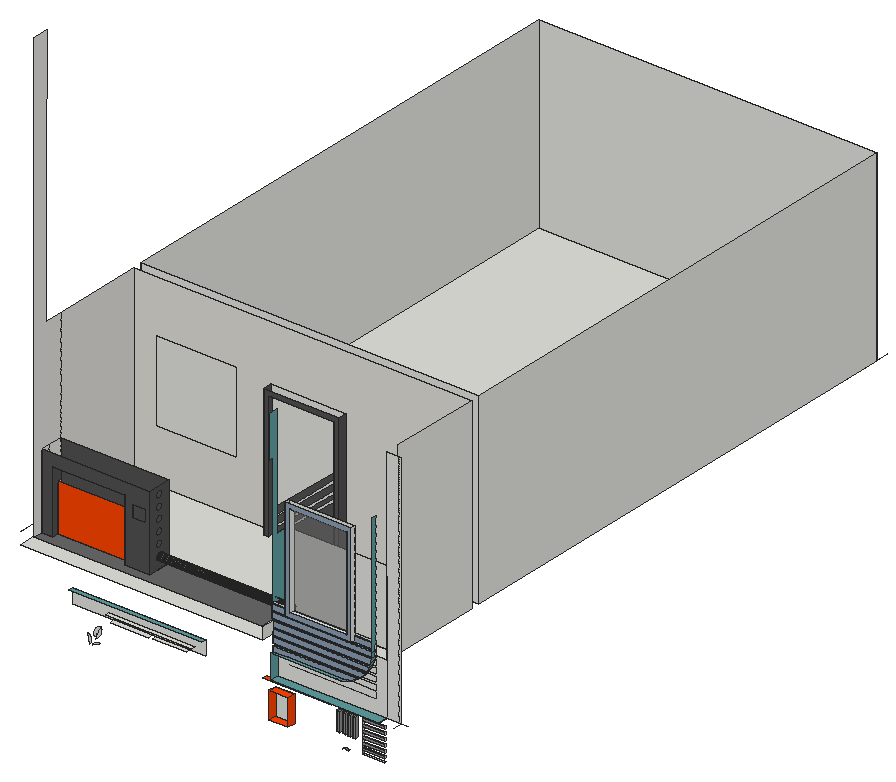
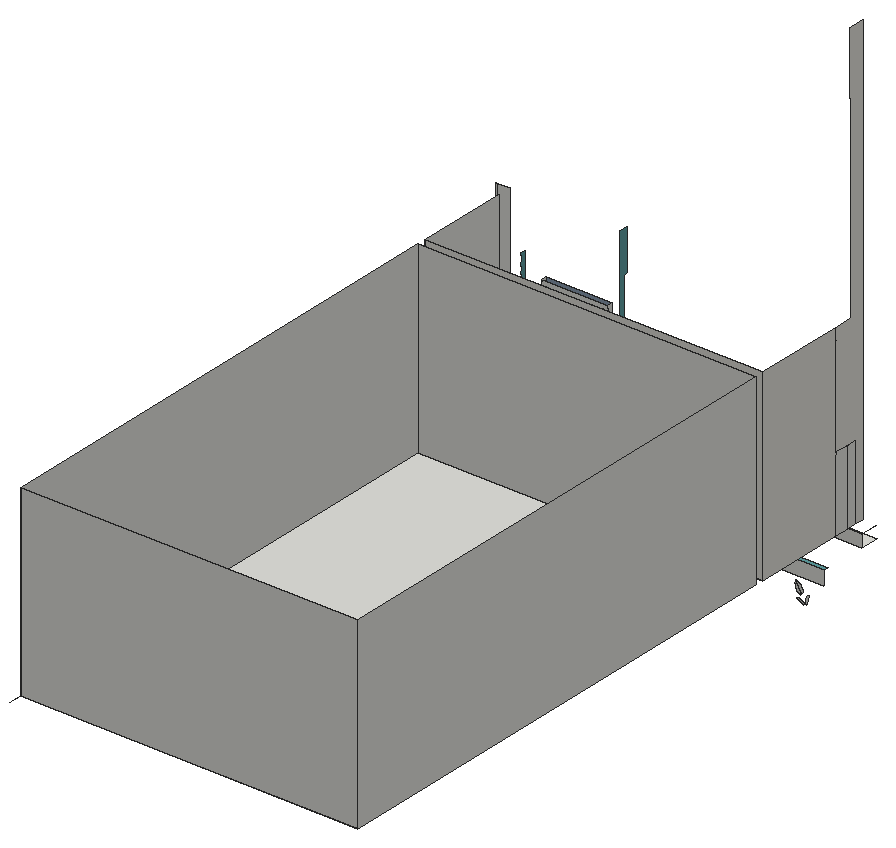
# SketchUp Ruby script. Lengths in inches.
U = 1.inch
M = Sketchup.active_model
def pt(a) = Geom::Point3d.new(a.map { |v| v * U })
def face(e, loops, mat)
  f = e.add_face(loops[0].map { |a| pt(a) })
  loops[1..].each { |l| e.add_face(l.map { |a| pt(a) }).erase! }
  f.material = f.back_material = mat if mat
  f
end
# faces: each face lists its corners as indices into pts; further lists are holes
def faces(e, pts, list, mat = nil) = list.each { |f| face(e, (f[0].is_a?(Array) ? f : [f]).map { |l| l.map { |i| pts[i] } }, mat) }
# xy, xz, yz: faces in a plane at the given z, y or x. An outline is a flat list of corners, or four numbers for a rectangle; further outlines are holes
def ring(l) = l.size == 4 ? [[l[0], l[1]], [l[2], l[1]], [l[2], l[3]], [l[0], l[3]]] : l.each_slice(2).to_a
def flat(e, list, mat, &to3) = list.each { |f| face(e, (f[0].is_a?(Array) ? f : [f]).map { |l| ring(l).map { |u, v| to3.(u, v) } }, mat) }
def xy(e, z, list, mat = nil) = flat(e, list, mat) { |x, y| [x, y, z] }
def xz(e, y, list, mat = nil) = flat(e, list, mat) { |x, z| [x, y, z] }
def yz(e, x, list, mat = nil) = flat(e, list, mat) { |y, z| [x, y, z] }
def lines(e, pts, list) = list.each { |a, b| e.add_line(pt(pts[a]), pt(pts[b])) }
# prism: a flat outline (further loops are holes) pulled along v
def prism(e, loops, v, mat = nil)
  f = face(e, loops, mat); d = Geom::Vector3d.new(v.map { |x| x * U })
  f.pushpull(f.normal.samedirection?(d) ? d.length : -d.length)
end
def box(e, o, s, mat = nil) = prism(e, [[o, [o[0] + s[0], o[1], o[2]], [o[0] + s[0], o[1] + s[1], o[2]], [o[0], o[1] + s[1], o[2]]]], [0, 0, s[2]], mat)
def at(x, y, z, deg = 0) = Geom::Transformation.translation(pt([x, y, z])) * Geom::Transformation.rotation(ORIGIN, Z_AXIS, deg.degrees)
def axes(o, x, y, z) = Geom::Transformation.new([*x, 0, *y, 0, *z, 0, *pt(o).to_a, 1])
def part(name) = M.definitions.add(name)
# library, detail: a bought-in or finely detailed component or shape, given as its bounding box
def library(name, o, s) = part(name).tap { |d| box(d.entities, o, s) }
def detail(e, o, s) = box(e.add_group.entities, o, s)
def put(e, d, t, mat = nil) = e.add_instance(d, t).tap { |i| i.material = mat if mat }
def group(e, t, mat = nil) = e.add_group.tap { |g| g.transformation = t; g.material = mat if mat }.entities
root = M.entities
M.materials.add("[0024_OrangeRed]").color = [255, 69, 0]
M.materials.add("[0081_CadetBlue]").color = [95, 158, 160]
M.materials.add("[0110_LightSlateGray]").color = [139, 158, 178]
M.materials.add("[0134_DimGray]").color = [105, 105, 105]
M.materials.add("[0135_DarkGray]").color = [81, 81, 81]
M.materials.add("[Color M04]").color = [142, 142, 142]
M.materials.add("[Marble Carrara Gold Floor Tile]").color = [225, 223, 217]
M.materials.add("[Translucent Glass Gray]").color = [128, 128, 128]
M.materials["[Translucent Glass Gray]"].alpha = 0.5
xy(root,61.1,[[216.37,11,230.7,12]])
xy(root,61.11,[[157.99,9,169.99,14.125]],"[0024_OrangeRed]")
xy(root,63.25,[[216.37,11,230.7,12]])
xy(root,64.54,[[216.37,11,230.7,12]])
xy(root,66.6875,[[216.37,11,230.7,12]])
xy(root,67.98,[[216.37,11,230.7,12]])
xy(root,69.76,[[211.55,9.125,213.55,11],[201.43,9.25,203.43,11],[204.8,9.25,206.8,11],[208.18,9.25,210.18,11]])
xy(root,70.125,[[216.37,11,230.7,12]])
xy(root,71.42,[[216.37,11,230.7,12]])
xy(root,73.5625,[[216.37,11,230.7,12]])
xy(root,74.85,[[216.37,11,230.7,12]])
xy(root,77,[[216.37,11,230.7,12]])
xy(root,78.23,[[157.99,9,169.99,14.125]],"[0024_OrangeRed]")
xy(root,78.29,[[216.37,11,230.7,12]])
xy(root,80.4375,[[216.37,11,230.7,12]])
xy(root,81.73,[[216.37,11,230.7,12]])
xy(root,81.89,[[211.55,9.125,213.55,11],[201.43,9.25,203.43,11],[204.8,9.25,206.8,11],[208.18,9.25,210.18,11]],"[Color M04]")
xy(root,83.5625,[[58.13,6,82.62,9],[85.26,6,107.11,9]])
xy(root,83.875,[[153.86,9,198.26,12]],"[0024_OrangeRed]")
xy(root,83.875,[[198.26,11,216.37,12]],"[Color M04]")
xy(root,86.5625,[[161.25,6,230.7,12]],"[0081_CadetBlue]")
xy(root,86.73,[[54.96,6,110.28,9]])
xy(root,90.99,[[29.19,9,114.82,12]],"[0081_CadetBlue]")
xy(root,102.07,[[161.25,6,203.39,9]],"[0081_CadetBlue]")
xy(root,102.24,[[161.25,8,170.69,9]])
xy(root,102.27,[[170.69,8,206.44,9]])
xy(root,105.62,[[161.25,8,215.65,9]],"[0110_LightSlateGray]")
xy(root,106.98,[[161.25,8,217.65,9]])
xy(root,110.36,[[161.25,8,221.11,9]],"[0110_LightSlateGray]")
xy(root,111.72,[[161.25,8,222.18,9]],"[0110_LightSlateGray]")
xy(root,112.3125,[[5,0,161.25,12]])
xy(root,115.1,[[161.25,8,224.19,9]],"[0110_LightSlateGray]")
xy(root,116.46,[[161.25,8,224.85,9]],"[0110_LightSlateGray]")
xy(root,116.6875,[[83.4375,12,160.53,21]])
xy(root,119.84,[[161.25,8,225.92,9]],"[0110_LightSlateGray]")
xy(root,120,[[160.53,0,161.25,9],[14,6,21.23,12],[67.5,6,83.4375,12],[160.53,9,161.25,12],[21.23,10.125,67.5,12],
  [14,12,83.4375,21],[160.53,12,231.375,21],[14,21,231.375,21,231.375,79.875,150.55,79.875,150.55,73.875,147.55,73.875,147.55,76.875,105.55,76.875,105.55,73.875,102.55,73.875,102.55,79.875,14,79.875],[102.55,73.875,105.55,73.875,105.55,76.875,147.55,76.875,147.55,73.875,150.55,73.875,150.55,79.875,102.55,79.875],[14,85.875,231.375,405.4375]])
xy(root,120,[[14,0,160.53,0,160.53,21,83.4375,21,83.4375,6,67.5,6,67.5,10.125,21.23,10.125,21.23,6,14,6]],"[0134_DimGray]")
xy(root,121.2,[[160.53,8,226.1875,9]],"[0110_LightSlateGray]")
xy(root,124.58,[[160.53,8,226.55,9]],"[0110_LightSlateGray]")
xy(root,125.95,[[160.53,8,226.59,9]],"[0110_LightSlateGray]")
xy(root,126.75,[[170.69,6,213.13,8],[170.69,8,213.13,9]])
xy(root,129.33,[[160.53,8,170.69,9],[213.13,8,226.59,9]],"[0110_LightSlateGray]")
xy(root,129.75,[[173.69,6,210.13,9]])
xz(root,6,[[[170.69,126.75,213.13,192.34],[173.69,129.75,210.13,189.37]]],"[0110_LightSlateGray]")
xz(root,6,[[[14,120,21.23,120,21.23,160.4375,67.5,160.4375,67.5,120,83.4375,120,83.4375,168,14,168],[72,148.91,81.25,157.04]]],"[0135_DarkGray]")
xz(root,8,[[161.25,102.24,170.69,102.24,170.69,102.27,206.44,102.27,209.4,102.86,212.27,103.83,214.99,105.17,215.65,105.62,161.25,105.62],[161.25,106.98,217.65,106.98,219.8,108.86,221.11,110.36,161.25,110.36],[161.25,111.72,222.18,111.72,223.48,113.66,224.19,115.1,161.25,115.1],[161.25,116.46,224.85,116.46,225.8,119.26,225.92,119.84,161.25,119.84],[160.53,121.2,226.1875,121.2,226.39,122.24,226.55,124.58,160.53,124.58],
  [160.53,125.95,226.59,125.95,226.59,129.33,213.13,129.33,213.13,126.75,170.69,126.75,170.69,129.33,160.53,129.33]],"[0110_LightSlateGray]")
xz(root,9,[[44.14,64.29,49.21,66.72,48.72,66.79,48.21,66.81,47.71,66.78,47.21,66.7,46.73,66.55,46.26,66.36,45.82,66.12,45.41,65.83,45.03,65.5,44.6875,65.13,44.39,64.73],[42.7,64.77,42.93,65.26,43.1,65.76,43.2,66.29,43.23,66.82,43.2,67.35,43.1,67.875,42.9375,68.38,42.71,68.87,42.42,69.32,42.08,69.73,41.69,70.09,41.26,70.4],[46.5,68.96,47.12,69.36,47.68,69.83,48.19,70.36,48.65,70.93,49.04,71.55,49.37,72.21,49.625,72.9,49.81,73.61,49.91,74.33,49.94,75.07,49.9,75.8,49.77,76.52,46.5,70.62,47.17,70.28],[45.41,70.12,45.84,70.96,46.5,70.62,49.77,76.52,49.06,76.38,48.37,76.14,47.72,75.8,47.125,75.38,46.6,74.875,46.14,74.3,45.78,73.67,45.5,73,45.33,72.29,45.25,71.5625,45.28,70.83],[161.25,102.07,203.39,102.07,206.42,102.26,206.44,102.27,170.69,102.27,170.69,102.24,161.25,102.24],
  [161.25,102.24,161.25,105.62,215.65,105.62,214.99,105.17,212.27,103.83,209.4,102.86,206.44,102.27,170.69,102.27,170.69,102.24],[213.13,102.24,226.59,102.24,226.59,105.62,215.65,105.62,214.99,105.17,212.27,103.83,209.4,102.86,206.44,102.27,213.13,102.27],[161.25,105.62,215.65,105.62,217.51,106.86,217.65,106.98,161.25,106.98],[161.25,106.98,161.25,110.36,221.11,110.36,219.8,108.86,217.65,106.98,213.13,106.98,213.13,107.01,170.69,107.01,170.69,106.98],[170.69,106.98,213.13,107.01],
  [217.65,106.98,226.59,106.98,226.59,110.36,221.11,110.36,219.8,108.86],[161.25,110.36,221.11,110.36,221.8,111.14,222.18,111.72,161.25,111.72],[161.25,111.72,161.25,115.1,224.19,115.1,223.48,113.66,222.18,111.72,213.13,111.72,213.13,111.75,170.69,111.75,170.69,111.72],[170.69,111.72,213.13,111.75],[222.18,111.72,226.59,111.72,226.59,115.1,224.19,115.1,223.48,113.66],
  [161.25,115.1,224.19,115.1,224.82,116.39,224.85,116.46,161.25,116.46],[160.53,116.46,161.25,119.84],[161.25,116.46,161.25,119.84,225.92,119.84,225.8,119.26,224.85,116.46,213.13,116.46,213.13,116.5,170.69,116.5,170.69,116.46],[170.69,116.46,213.13,116.5],[224.85,116.46,226.59,116.46,226.59,119.84,225.92,119.84,225.8,119.26],
  [161.25,119.84,225.92,119.84,226.1875,121.2,160.53,121.2,160.53,120,161.25,120],[160.53,121.2,160.53,124.58,226.55,124.58,226.39,122.24,226.1875,121.2,213.13,121.2,213.13,121.24,170.69,121.24,170.69,121.2],[170.69,121.2,213.13,121.24],[226.1875,121.2,226.59,121.2,226.59,124.58,226.55,124.58,226.39,122.24],[160.53,124.58,226.55,124.58,226.59,125.26,226.59,125.95,160.53,125.95],
  [160.53,125.95,160.53,129.33,170.69,129.33,170.69,126.75,213.13,126.75,213.13,129.33,226.59,129.33,226.59,125.95,213.13,125.95,213.13,125.98,170.69,125.98,170.69,125.95],[170.69,125.95,213.13,125.98],[[170.69,126.75,213.13,192.34],[173.69,129.75,210.13,189.37]],[160.53,129.33,170.69,130.6875],[213.13,129.33,226.59,130.6875]])
xz(root,9,[[173.69,129.75,210.13,189.37]],"[Translucent Glass Gray]")
xz(root,9.125,[[211.55,69.76,213.55,81.89]],"[Color M04]")
xz(root,9.25,[[201.43,69.76,203.43,81.89],[204.8,69.76,206.8,81.89],[208.18,69.76,210.18,81.89]],"[Color M04]")
xz(root,10.125,[[21.23,120,67.5,150.3]],"[0024_OrangeRed]")
xz(root,11,[[216.37,63.25,230.7,64.54],[216.37,66.6875,230.7,67.98],[216.37,70.125,230.7,71.42],[216.37,73.5625,230.7,74.85],[216.37,77,230.7,78.29],
  [216.37,80.4375,230.7,81.73]],"[Color M04]")
xz(root,12,[[29.19,81.74,114.82,90.99],[161.25,86.5625,231.375,120],[231.375,86.5625,238.75,240],[238.75,86.5625,240.375,240],[5,112.3125,5,120,83.4375,120,83.4375,116.6875,160.53,116.6875,160.53,120,161.25,120,161.25,112.3125]])
xz(root,14.125,[[157.99,61.11,169.99,78.23]])
xz(root,21,[[83.4375,116.6875,160.53,120],[160.53,120,231.375,168]])
xz(root,21,[[14,120,83.4375,168]],"[0135_DarkGray]")
xz(root,73.875,[[102.55,120,105.55,120,105.55,201,147.55,201,147.55,120,150.55,120,150.55,204,102.55,204]],"[0135_DarkGray]")
xz(root,76.875,[[105.55,118.21,107.61,120,106.51,120,105.55,119.14],[106.51,120,107.61,120,147.55,154.73,147.55,156.46],[105.55,122.71,147.55,159.23,147.55,160.96,105.55,123.64],[105.55,128.71,147.55,165.23,147.55,166.96,105.55,129.64]])
xz(root,76.875,[[105.55,120,106.51,120,147.55,156.46,147.55,159.23,105.55,122.71],[107.61,120,147.55,120,147.55,154.73],[105.55,123.64,147.55,160.96,147.55,165.23,105.55,128.71],[105.55,129.64,147.55,166.96,147.55,171.23,105.55,134.71]],"[0135_DarkGray]")
xz(root,79.875,[[102.55,120,150.55,204]])
xz(root,79.875,[[[14,120,102.55,120,102.55,204,150.55,204,150.55,120,231.375,120,231.375,240,14,240],[28.3,153.81,80.67,206.18]]],"[Marble Carrara Gold Floor Tile]")
xz(root,85.875,[[14,120,231.375,240]])
xz(root,405.4375,[[14,120,231.375,240]])
yz(root,14,[[6,120,12,168],[12,120,21,168],[85.875,120,405.4375,240]])
yz(root,14,[[0,120,6,120,6,168,21,168,21,240,9,240,9,367.625,10.4375,367.625,10.4375,407.79,0,407.79],[21,120,79.875,240]],"[Marble Carrara Gold Floor Tile]")
yz(root,21.23,[[10.125,120,12,150.3]])
yz(root,21.23,[[6,120,10.125,120,10.125,150.3,12,150.3,12,160.4375,6,160.4375]],"[0135_DarkGray]")
yz(root,67.5,[[10.125,120,12,150.3]])
yz(root,67.5,[[6,120,6,160.4375,12,160.4375,12,150.3,10.125,150.3,10.125,120]],"[0135_DarkGray]")
yz(root,83.4375,[[12,116.6875,21,120]])
yz(root,83.4375,[[[6,120,21,168],[13.48,160.8125,12.89,160.89,12.35,161.11,11.88,161.47,11.53,161.9375,11.3,162.48,11.23,163.0625,11.3,163.64,11.53,164.1875,11.88,164.65,12.35,165.01,12.89,165.23,13.48,165.3125,14.06,165.23,14.6,165.01,15.07,164.65,15.42,164.1875,15.65,163.64,15.73,163.0625,15.65,162.48,15.42,161.9375,15.07,161.47,14.6,161.11,14.06,160.89],[13.48,153.6875,12.89,153.76,12.35,153.99,11.88,154.34,11.53,154.8125,11.3,155.35,11.23,155.9375,11.3,156.52,11.53,157.0625,11.88,157.53,12.35,157.88,12.89,158.11,13.48,158.1875,14.06,158.11,14.6,157.88,15.07,157.53,15.42,157.0625,15.65,156.52,15.73,155.9375,15.65,155.35,15.42,154.8125,15.07,154.34,14.6,153.99,14.06,153.76],[13.48,146.5625,12.89,146.64,12.35,146.86,11.88,147.22,11.53,147.6875,11.3,148.23,11.23,148.8125,11.3,149.39,11.53,149.9375,11.88,150.4,12.35,150.76,12.89,150.98,13.48,151.0625,14.06,150.98,14.6,150.76,15.07,150.4,15.42,149.9375,15.65,149.39,15.73,148.8125,15.65,148.23,15.42,147.6875,15.07,147.22,14.6,146.86,14.06,146.64],[13.48,139.4375,12.89,139.51,12.35,139.74,11.88,140.09,11.53,140.5625,11.3,141.1,11.23,141.6875,11.3,142.27,11.53,142.8125,11.88,143.28,12.35,143.63,12.89,143.86,13.48,143.9375,14.06,143.86,14.6,143.63,15.07,143.28,15.42,142.8125,15.65,142.27,15.73,141.6875,15.65,141.1,15.42,140.5625,15.07,140.09,14.6,139.74,14.06,139.51],[13.48,132.3125,12.89,132.39,12.35,132.61,11.88,132.97,11.53,133.4375,11.3,133.98,11.23,134.5625,11.3,135.14,11.53,135.6875,11.88,136.15,12.35,136.51,12.89,136.73,13.48,136.8125,14.06,136.73,14.6,136.51,15.07,136.15,15.42,135.6875,15.65,135.14,15.73,134.5625,15.65,133.98,15.42,133.4375,15.07,132.97,14.6,132.61,14.06,132.39],[13.48,125.1875,12.89,125.26,12.35,125.49,11.88,125.84,11.53,126.3125,11.3,126.85,11.23,127.4375,11.3,128.02,11.53,128.5625,11.88,129.03,12.35,129.38,12.89,129.61,13.48,129.6875,14.06,129.61,14.6,129.38,15.07,129.03,15.42,128.5625,15.65,128.02,15.73,127.4375,15.65,126.85,15.42,126.3125,15.07,125.84,14.6,125.49,14.06,125.26]]],"[0135_DarkGray]")
yz(root,102.55,[[73.875,120,79.875,204]],"[0135_DarkGray]")
yz(root,105.55,[[73.875,120,76.875,201]],"[0135_DarkGray]")
yz(root,147.55,[[73.875,120,76.875,201]],"[0135_DarkGray]")
yz(root,150.55,[[73.875,120,79.875,204]],"[0135_DarkGray]")
yz(root,157.99,[[9,61.11,14.125,78.23]],"[0024_OrangeRed]")
yz(root,160.53,[[12,116.6875,21,120]])
yz(root,160.53,[[9,120,9,213.14,6,213.14,6,240,12,240,12,168,21,168,21,120]],"[0081_CadetBlue]")
yz(root,160.53,[[8,121.2,9,124.58],[8,125.95,9,129.33]],"[0110_LightSlateGray]")
yz(root,161.25,[[8,102.24,9,105.62],[8,106.98,9,110.36],[8,111.72,9,112.3125],[0,112.3125,8,112.3125,8,115.1,9,115.1,9,116.46,8,116.46,8,119.84,9,119.84,9,120,0,120],[8,112.3125,9,115.1],
  [9,112.3125,12,120],[8,116.46,9,119.84]])
yz(root,161.25,[[6,86.5625,6,102.07,9,102.07,9,112.3125,12,112.3125,12,86.5625]],"[0081_CadetBlue]")
yz(root,169.375,[[13.48,125.1875,14.06,125.26,14.6,125.49,15.07,125.84,15.42,126.3125,15.65,126.85,15.73,127.4375,15.65,128.02,15.42,128.5625,15.07,129.03,14.6,129.38,14.06,129.61,13.48,129.6875,12.89,129.61,12.35,129.38,11.88,129.03,11.53,128.5625,11.3,128.02,11.23,127.4375,11.3,126.85,11.53,126.3125,11.88,125.84,12.35,125.49,12.89,125.26]])
yz(root,169.99,[[9,61.11,14.125,78.23]],"[0024_OrangeRed]")
yz(root,170.69,[[8,102.24,9,102.27],[6,126.75,6,192.34,9,192.34,9,190.98,8,190.98,8,187.59,9,187.59,9,186.23,8,186.23,8,182.85,9,182.85,9,181.49,8,181.49,8,178.11,9,178.11,9,176.75,8,176.75,8,173.37,9,173.37,9,172.01,8,172.01,8,168.625,9,168.625,9,167.26,8,167.26,8,163.88,9,163.88,9,162.52,8,162.52,8,159.14,9,159.14,9,157.78,8,157.78,8,154.4,9,154.4,9,153.04,8,153.04,8,149.66,9,149.66,9,148.3,8,148.3,8,144.92,9,144.92,9,143.55,8,143.55,8,140.17,9,140.17,9,138.8125,8,138.8125,8,135.43,9,135.43,9,134.07,8,134.07,8,130.6875,9,130.6875,9,129.33,8,129.33,8,126.75],[8,126.75,9,129.33]])
yz(root,173.69,[[6,129.75,9,189.37]])
yz(root,201.43,[[9.25,69.76,11,81.89]],"[Color M04]")
yz(root,203.43,[[9.25,69.76,11,81.89]],"[Color M04]")
yz(root,204.8,[[9.25,69.76,11,81.89]],"[Color M04]")
yz(root,206.8,[[9.25,69.76,11,81.89]],"[Color M04]")
yz(root,208.18,[[9.25,69.76,11,81.89]],"[Color M04]")
yz(root,210.13,[[6,129.75,9,189.37]])
yz(root,210.18,[[9.25,69.76,11,81.89]],"[Color M04]")
yz(root,211.55,[[9.125,69.76,11,81.89]],"[Color M04]")
yz(root,213.13,[[6,126.75,8,126.75,8,129.33,9,129.33,9,130.6875,8,130.6875,8,134.07,9,134.07,9,135.43,8,135.43,8,138.8125,9,138.8125,9,140.17,8,140.17,8,143.55,9,143.55,9,144.92,8,144.92,8,148.3,9,148.3,9,149.66,8,149.66,8,153.04,9,153.04,9,154.4,8,154.4,8,157.78,9,157.78,9,159.14,8,159.14,8,162.52,9,162.52,9,163.88,8,163.88,8,167.26,9,167.26,9,168.625,8,168.625,8,172.01,9,172.01,9,173.37,8,173.37,8,176.75,9,176.75,9,178.11,8,178.11,8,181.49,9,181.49,9,182.85,8,182.85,8,186.23,9,186.23,9,187.59,8,187.59,8,190.98,9,190.98,9,192.34,6,192.34],[8,126.75,9,129.33]])
yz(root,213.55,[[9.125,69.76,11,81.89]],"[Color M04]")
yz(root,216.37,[[11,67.98,12,70.125],[11,71.42,12,73.5625],[11,74.85,12,77],[11,78.29,12,80.4375],[11,81.73,12,83.875]])
yz(root,216.37,[[11,61.1,12,63.25],[11,64.54,12,66.6875]],"[Color M04]")
yz(root,226.59,[[8,125.95,9,129.33]])
yz(root,226.59,[[6,125.26,6,202.88,9,202.88,9,201.62,8,201.62,8,197.1,9,197.1,9,195.72,8,195.72,8,192.34,9,192.34,9,190.98,8,190.98,8,187.59,9,187.59,9,186.23,8,186.23,8,182.85,9,182.85,9,181.49,8,181.49,8,178.11,9,178.11,9,176.75,8,176.75,8,173.37,9,173.37,9,172.01,8,172.01,8,168.625,9,168.625,9,167.26,8,167.26,8,163.88,9,163.88,9,162.52,8,162.52,8,159.14,9,159.14,9,157.78,8,157.78,8,154.4,9,154.4,9,153.04,8,153.04,8,149.66,9,149.66,9,148.3,8,148.3,8,144.92,9,144.92,9,143.55,8,143.55,8,140.17,9,140.17,9,138.8125,8,138.8125,8,135.43,9,135.43,9,134.07,8,134.07,8,130.6875,9,130.6875,9,129.33,8,129.33,8,125.95,9,125.95,9,125.26]],"[0081_CadetBlue]")
yz(root,230.7,[[11,63.25,12,64.54],[11,66.6875,12,67.98],[11,70.125,12,71.42],[11,73.5625,12,74.85],[11,77,12,78.29],
  [11,80.4375,12,81.73]])
yz(root,231.375,[[12,120,21,168],[21,120,79.875,240],[85.875,120,405.4375,240]])
p = [[205.47,11,61.03],[204.65,11,60.6875],[204.65,10,60.6875],[205.47,10,61.03],[208.03,11,60.6875],[207.21,11,61.03],
  [207.21,10,61.03],[208.03,10,60.6875],[206.34,11,61.14],[206.34,10,61.14],[206.42,9,102.26],[203.39,9,102.07],
  [203.39,6,102.07],[206.42,6,102.26],[206.44,9,102.27],[209.4,6,102.86],[209.4,8,102.86],[206.44,8,102.27],
  [209.4,9,102.86],[212.27,6,103.83],[212.27,8,103.83],[212.27,9,103.83],[214.99,6,105.17],[214.99,8,105.17],
  [214.99,9,105.17],[217.51,9,106.86],[215.65,9,105.62],[215.65,8,105.62],[217.51,6,106.86],[217.65,9,106.98],
  [219.8,6,108.86],[219.8,8,108.86],[217.65,8,106.98],[219.8,9,108.86],[221.8,9,111.14],[221.11,9,110.36],
  [221.11,8,110.36],[221.8,6,111.14],[222.18,9,111.72],[223.48,6,113.66],[223.48,8,113.66],[222.18,8,111.72],
  [223.48,9,113.66],[224.82,9,116.39],[224.19,9,115.1],[224.19,8,115.1],[224.82,6,116.39],[224.85,9,116.46],
  [225.8,6,119.26],[225.8,8,119.26],[224.85,8,116.46],[225.8,9,119.26],[226.1875,9,121.2],[225.92,9,119.84],
  [225.92,8,119.84],[226.39,6,122.24],[226.39,8,122.24],[226.1875,8,121.2],[226.39,9,122.24],[226.59,9,125.26],
  [226.55,9,124.58],[226.55,8,124.58],[226.59,6,125.26],[83.4375,12.89,125.26],[83.4375,13.48,125.1875],[169.375,13.48,125.1875],
  [169.375,12.89,125.26],[83.4375,14.06,125.26],[169.375,14.06,125.26],[83.4375,12.35,125.49],[169.375,12.35,125.49],[83.4375,14.6,125.49],
  [169.375,14.6,125.49],[83.4375,11.88,125.84],[169.375,11.88,125.84],[83.4375,15.07,125.84],[169.375,15.07,125.84],[83.4375,11.53,126.3125],
  [169.375,11.53,126.3125],[83.4375,15.42,126.3125],[169.375,15.42,126.3125],[83.4375,11.3,126.85],[169.375,11.3,126.85],[83.4375,15.65,126.85],
  [169.375,15.65,126.85],[83.4375,11.23,127.4375],[169.375,11.23,127.4375],[83.4375,15.73,127.4375],[169.375,15.73,127.4375],[83.4375,11.3,128.02],
  [169.375,11.3,128.02],[83.4375,15.65,128.02],[169.375,15.65,128.02],[83.4375,11.53,128.5625],[169.375,11.53,128.5625],[83.4375,15.42,128.5625],
  [169.375,15.42,128.5625],[83.4375,11.88,129.03],[169.375,11.88,129.03],[83.4375,15.07,129.03],[169.375,15.07,129.03],[83.4375,12.35,129.38],
  [169.375,12.35,129.38],[83.4375,14.6,129.38],[169.375,14.6,129.38],[83.4375,12.89,129.61],[169.375,12.89,129.61],[83.4375,14.06,129.61],
  [169.375,14.06,129.61],[83.4375,13.48,129.6875],[169.375,13.48,129.6875],[231.375,405.4375,120],[231.375,414.4375,120],[161.25,9,115.1],
  [160.53,9,115.1],[213.13,9,97.49],[213.13,9,97.53],[226.59,9,100.875],[226.59,9,97.49],[170.69,9,97.53],
  [170.69,9,97.49],[170.69,8,107.01],[170.69,8,106.98],[170.69,8,111.75],[170.69,8,111.72],[170.69,8,116.5],
  [170.69,8,116.46],[170.69,8,121.24],[170.69,8,121.2],[170.69,8,125.98],[170.69,8,125.95],[231.375,12,86.5625],
  [231.375,6,86.5625],[240.375,12,86.5625],[240.375,6,86.5625],[245.1875,12,86.5625],[5,12,120],[5,0,120]]
faces(root,p,[[0,1,2,3],[4,5,6,7],[8,0,3,9],[5,8,9,6]],"[Color M04]")
faces(root,p,[[10,11,12,13],[14,10,13,15,16,17],[19,20,16,15],[22,23,20,19],[25,26,27,23,22,28],[29,25,28,30,31,32],[34,35,36,31,30,37],[38,34,37,39,40,41],
  [43,44,45,40,39,46],[47,43,46,48,49,50],[52,53,54,49,48,55,56,57],[59,60,61,56,55,62]],"[0081_CadetBlue]")
faces(root,p,[[18,14,17,16],[21,18,16,20],[24,21,20,23],[26,24,23,27],[33,29,32,31],[35,33,31,36],[42,38,41,40],[44,42,40,45],
  [51,47,50,49],[53,51,49,54],[58,52,57,56],[60,58,56,61]])
faces(root,p,[[63,64,65,66],[64,67,68,65],[69,63,66,70],[67,71,72,68],[73,69,70,74],[71,75,76,72],[77,73,74,78],[75,79,80,76],
  [81,77,78,82],[79,83,84,80],[85,81,82,86],[83,87,88,84],[89,85,86,90],[87,91,92,88],[93,89,90,94],[91,95,96,92],
  [97,93,94,98],[95,99,100,96],[101,97,98,102],[99,103,104,100],[105,101,102,106],[103,107,108,104],[109,105,106,110],[107,109,110,108]],"[0134_DimGray]")
lines(root,p,[[111,112],[113,114],[115,116],[117,118],[115,118],[119,120],[116,119],[121,122],[123,124],[125,126],[127,128],[129,130],
  [131,132],[133,134],[133,135],[136,137]])
